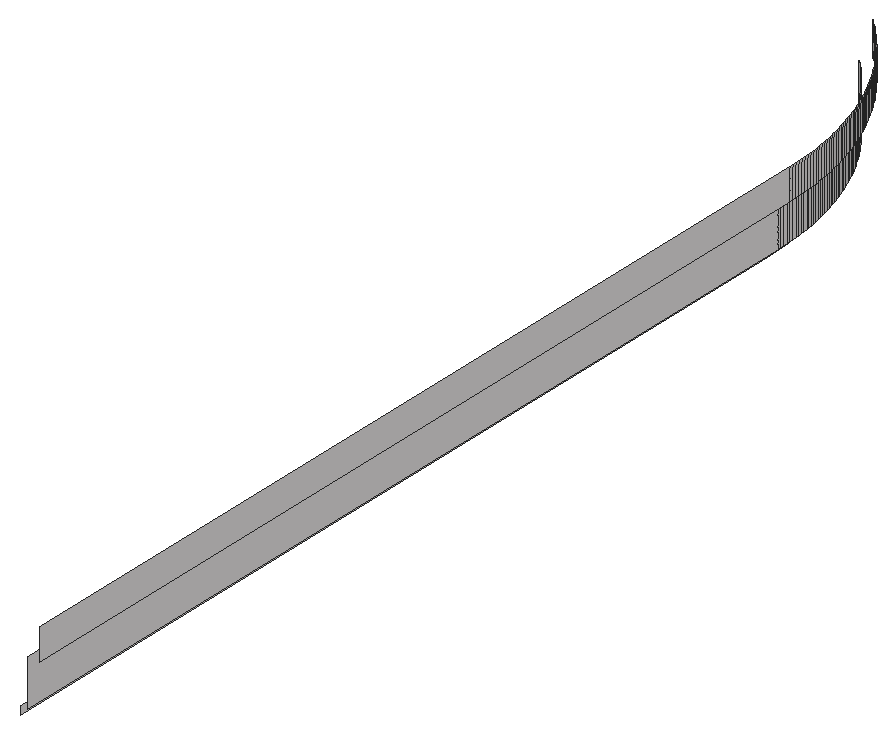
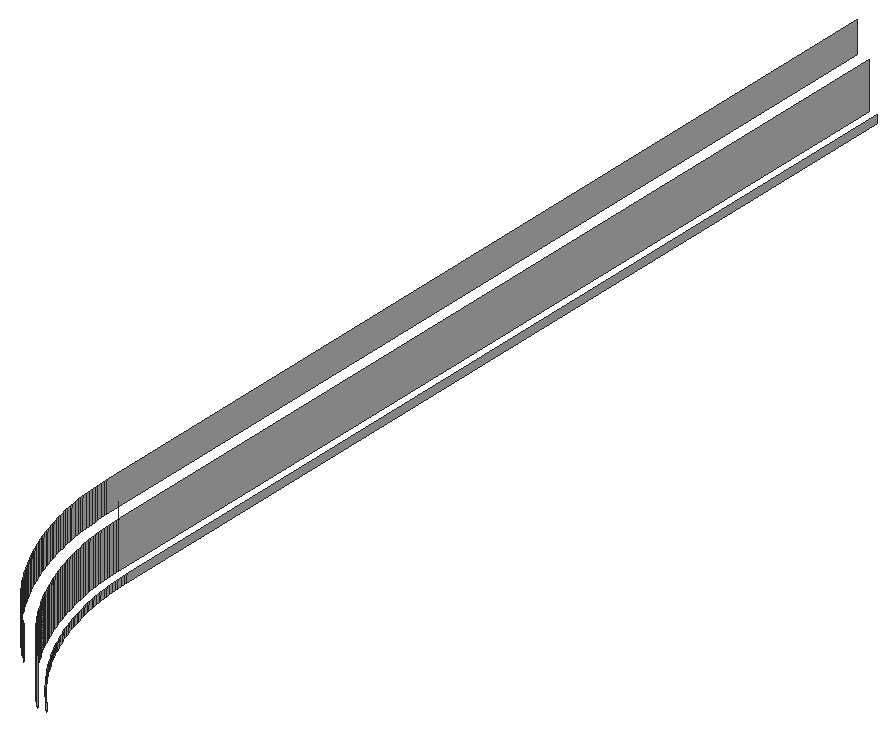
# SketchUp Ruby script. Lengths in inches.
U = 1.inch
M = Sketchup.active_model
def pt(a) = Geom::Point3d.new(a.map { |v| v * U })
def face(e, loops, mat)
  f = e.add_face(loops[0].map { |a| pt(a) })
  loops[1..].each { |l| e.add_face(l.map { |a| pt(a) }).erase! }
  f.material = f.back_material = mat if mat
  f
end
# faces: each face lists its corners as indices into pts; further lists are holes
def faces(e, pts, list, mat = nil) = list.each { |f| face(e, (f[0].is_a?(Array) ? f : [f]).map { |l| l.map { |i| pts[i] } }, mat) }
# xy, xz, yz: faces in a plane at the given z, y or x. An outline is a flat list of corners, or four numbers for a rectangle; further outlines are holes
def ring(l) = l.size == 4 ? [[l[0], l[1]], [l[2], l[1]], [l[2], l[3]], [l[0], l[3]]] : l.each_slice(2).to_a
def flat(e, list, mat, &to3) = list.each { |f| face(e, (f[0].is_a?(Array) ? f : [f]).map { |l| ring(l).map { |u, v| to3.(u, v) } }, mat) }
def xy(e, z, list, mat = nil) = flat(e, list, mat) { |x, y| [x, y, z] }
def xz(e, y, list, mat = nil) = flat(e, list, mat) { |x, z| [x, y, z] }
def yz(e, x, list, mat = nil) = flat(e, list, mat) { |y, z| [x, y, z] }
def lines(e, pts, list) = list.each { |a, b| e.add_line(pt(pts[a]), pt(pts[b])) }
# prism: a flat outline (further loops are holes) pulled along v
def prism(e, loops, v, mat = nil)
  f = face(e, loops, mat); d = Geom::Vector3d.new(v.map { |x| x * U })
  f.pushpull(f.normal.samedirection?(d) ? d.length : -d.length)
end
def box(e, o, s, mat = nil) = prism(e, [[o, [o[0] + s[0], o[1], o[2]], [o[0] + s[0], o[1] + s[1], o[2]], [o[0], o[1] + s[1], o[2]]]], [0, 0, s[2]], mat)
def at(x, y, z, deg = 0) = Geom::Transformation.translation(pt([x, y, z])) * Geom::Transformation.rotation(ORIGIN, Z_AXIS, deg.degrees)
def axes(o, x, y, z) = Geom::Transformation.new([*x, 0, *y, 0, *z, 0, *pt(o).to_a, 1])
def part(name) = M.definitions.add(name)
# library, detail: a bought-in or finely detailed component or shape, given as its bounding box
def library(name, o, s) = part(name).tap { |d| box(d.entities, o, s) }
def detail(e, o, s) = box(e.add_group.entities, o, s)
def put(e, d, t, mat = nil) = e.add_instance(d, t).tap { |i| i.material = mat if mat }
def group(e, t, mat = nil) = e.add_group.tap { |g| g.transformation = t; g.material = mat if mat }.entities
root = M.entities
M.materials.add("[Quartz Light Brown]").color = [215, 212, 212]
yz(root,501,[[320.7,486,440.7,487],[440.7,486,441.19,487]],"[Quartz Light Brown]")
yz(root,502,[[320.7,487,440.7,493],[440.7,487,441.2,493]],"[Quartz Light Brown]")
yz(root,503.5,[[320.7,493,440.7,497],[440.7,493,441.22,497]],"[Quartz Light Brown]")
p = [[501,441.19,486],[500.99,441.67,486],[500.99,441.67,487],[501,441.19,487],[500.97,442.15,486],[500.97,442.15,487],
  [500.95,442.64,486],[500.95,442.64,487],[500.92,443.12,486],[500.92,443.12,487],[500.89,443.6,486],[500.89,443.6,487],
  [500.84,444.09,486],[500.84,444.09,487],[500.8,444.57,486],[500.8,444.57,487],[500.74,445.05,486],[500.74,445.05,487],
  [500.68,445.53,486],[500.68,445.53,487],[500.62,446.01,486],[500.62,446.01,487],[500.54,446.49,486],[500.54,446.49,487],
  [500.47,446.97,486],[500.47,446.97,487],[500.38,447.44,486],[500.38,447.44,487],[500.29,447.92,486],[500.29,447.92,487],
  [500.19,448.39,486],[500.19,448.39,487],[500.09,448.87,486],[500.09,448.87,487],[499.98,449.34,486],[499.98,449.34,487],
  [499.86,449.81,486],[499.86,449.81,487],[499.74,450.28,486],[499.74,450.28,487],[499.61,450.74,486],[499.61,450.74,487],
  [499.48,451.21,486],[499.48,451.21,487],[499.34,451.67,486],[499.34,451.67,487],[499.1875,452.13,486],[499.1875,452.13,487],
  [499.04,452.59,486],[499.04,452.59,487],[498.88,453.05,486],[498.88,453.05,487],[498.71,453.51,486],[498.71,453.51,487],
  [498.54,453.96,486],[498.54,453.96,487],[498.37,454.41,486],[498.37,454.41,487],[498.18,454.86,486],[498.18,454.86,487],
  [498,455.31,486],[498,455.31,487],[497.8,455.75,486],[497.8,455.75,487],[497.6,456.19,486],[497.6,456.19,487],
  [497.4,456.63,486],[497.4,456.63,487],[497.18,457.07,486],[497.18,457.07,487],[496.97,457.5,486],[496.97,457.5,487],
  [496.74,457.93,486],[496.74,457.93,487],[496.52,458.36,486],[496.52,458.36,487],[496.28,458.78,486],[496.28,458.78,487],
  [496.04,459.2,486],[496.04,459.2,487],[495.8,459.62,486],[495.8,459.62,487],[495.55,460.03,486],[495.55,460.03,487],
  [495.29,460.44,486],[495.29,460.44,487],[495.03,460.85,486],[495.03,460.85,487],[494.76,461.26,486],[494.76,461.26,487],
  [494.49,461.66,486],[494.49,461.66,487],[494.22,462.06,486],[494.22,462.06,487],[493.93,462.45,486],[493.93,462.45,487],
  [493.65,462.84,486],[493.65,462.84,487],[493.35,463.23,486],[493.35,463.23,487],[493.06,463.61,486],[493.06,463.61,487],
  [492.75,463.99,486],[492.75,463.99,487],[492.45,464.36,486],[492.45,464.36,487],[492.14,464.73,486],[492.14,464.73,487],
  [491.82,465.1,486],[491.82,465.1,487],[491.5,465.46,486],[491.5,465.46,487],[491.17,465.82,486],[491.17,465.82,487],
  [490.84,466.17,486],[490.84,466.17,487],[501.99,441.7,487],[501.99,441.7,493],[502,441.2,493],[502,441.2,487],
  [501.97,442.19,487],[501.97,442.19,493],[501.95,442.69,487],[501.95,442.69,493],[501.92,443.1875,487],[501.92,443.1875,493],
  [501.88,443.68,487],[501.88,443.68,493],[501.84,444.18,487],[501.84,444.18,493],[501.79,444.67,487],[501.79,444.67,493],
  [501.74,445.17,487],[501.74,445.17,493],[501.67,445.66,487],[501.67,445.66,493],[501.61,446.15,487],[501.61,446.15,493],
  [501.53,446.65,487],[501.53,446.65,493],[501.45,447.14,487],[501.45,447.14,493],[501.36,447.625,487],[501.36,447.625,493],
  [501.27,448.11,487],[501.27,448.11,493],[501.17,448.6,487],[501.17,448.6,493],[501.0625,449.09,487],[501.0625,449.09,493],
  [500.95,449.57,487],[500.95,449.57,493],[500.83,450.05,487],[500.83,450.05,493],[500.71,450.54,487],[500.71,450.54,493],
  [500.57,451.02,487],[500.57,451.02,493],[500.44,451.49,487],[500.44,451.49,493],[500.29,451.97,487],[500.29,451.97,493],
  [500.14,452.44,487],[500.14,452.44,493],[499.98,452.92,487],[499.98,452.92,493],[499.82,453.39,487],[499.82,453.39,493],
  [499.65,453.85,487],[499.65,453.85,493],[499.48,454.32,487],[499.48,454.32,493],[499.29,454.78,487],[499.29,454.78,493],
  [499.11,455.24,487],[499.11,455.24,493],[498.91,455.7,487],[498.91,455.7,493],[498.71,456.16,487],[498.71,456.16,493],
  [498.51,456.61,487],[498.51,456.61,493],[498.3,457.06,487],[498.3,457.06,493],[498.08,457.51,487],[498.08,457.51,493],
  [497.86,457.95,487],[497.86,457.95,493],[497.63,458.39,487],[497.63,458.39,493],[497.4,458.83,487],[497.4,458.83,493],
  [497.15,459.27,487],[497.15,459.27,493],[496.91,459.7,487],[496.91,459.7,493],[496.66,460.13,487],[496.66,460.13,493],
  [496.4,460.56,487],[496.4,460.56,493],[496.14,460.98,487],[496.14,460.98,493],[495.87,461.4,487],[495.87,461.4,493],
  [495.6,461.8125,487],[495.6,461.8125,493],[495.32,462.22,487],[495.32,462.22,493],[495.03,462.63,487],[495.03,462.63,493],
  [494.74,463.04,487],[494.74,463.04,493],[494.45,463.4375,487],[494.45,463.4375,493],[494.15,463.83,487],[494.15,463.83,493],
  [493.84,464.23,487],[493.84,464.23,493],[493.53,464.62,487],[493.53,464.62,493],[493.22,465,487],[493.22,465,493],
  [492.9,465.38,487],[492.9,465.38,493],[492.57,465.76,487],[492.57,465.76,493],[492.24,466.13,487],[492.24,466.13,493],
  [491.9,466.5,487],[491.9,466.5,493],[491.5625,466.86,487],[491.5625,466.86,493],[491.22,467.22,487],[491.22,467.22,493],
  [490.87,467.57,487],[490.87,467.57,493],[503.5,441.22,493],[503.49,441.73,493],[503.49,441.73,497],[503.5,441.22,497],
  [503.47,442.25,493],[503.47,442.25,497],[503.45,442.77,493],[503.45,442.77,497],[503.42,443.28,493],[503.42,443.28,497],
  [503.38,443.8,493],[503.38,443.8,497],[503.33,444.32,493],[503.33,444.32,497],[503.28,444.83,493],[503.28,444.83,497],
  [503.23,445.34,493],[503.23,445.34,497],[503.16,445.86,493],[503.16,445.86,497],[503.09,446.37,493],[503.09,446.37,497],
  [503.01,446.88,493],[503.01,446.88,497],[502.93,447.39,493],[502.93,447.39,497],[502.84,447.9,493],[502.84,447.9,497],
  [502.74,448.41,493],[502.74,448.41,497],[502.64,448.91,493],[502.64,448.91,497],[502.53,449.42,493],[502.53,449.42,497],
  [502.41,449.92,493],[502.41,449.92,497],[502.28,450.42,493],[502.28,450.42,497],[502.15,450.92,493],[502.15,450.92,497],
  [502.02,451.42,493],[502.02,451.42,497],[501.875,451.92,493],[501.875,451.92,497],[501.72,452.41,493],[501.72,452.41,497],
  [501.57,452.91,493],[501.57,452.91,497],[501.4,453.4,493],[501.4,453.4,497],[501.23,453.89,493],[501.23,453.89,497],
  [501.06,454.37,493],[501.06,454.37,497],[500.875,454.86,493],[500.875,454.86,497],[500.6875,455.34,493],[500.6875,455.34,497],
  [500.49,455.82,493],[500.49,455.82,497],[500.29,456.29,493],[500.29,456.29,497],[500.09,456.77,493],[500.09,456.77,497],
  [499.87,457.24,493],[499.87,457.24,497],[499.65,457.71,493],[499.65,457.71,497],[499.43,458.17,493],[499.43,458.17,497],
  [499.19,458.63,493],[499.19,458.63,497],[498.96,459.09,493],[498.96,459.09,497],[498.71,459.55,493],[498.71,459.55,497],
  [498.46,460,493],[498.46,460,497],[498.21,460.45,493],[498.21,460.45,497],[497.95,460.9,493],[497.95,460.9,497],
  [497.68,461.34,493],[497.68,461.34,497],[497.41,461.78,493],[497.41,461.78,497],[497.13,462.21,493],[497.13,462.21,497],
  [496.84,462.65,493],[496.84,462.65,497],[496.55,463.07,493],[496.55,463.07,497],[496.26,463.5,493],[496.26,463.5,497],
  [495.96,463.92,493],[495.96,463.92,497],[495.65,464.33,493],[495.65,464.33,497],[495.34,464.75,493],[495.34,464.75,497],
  [495.02,465.16,493],[495.02,465.16,497],[494.7,465.56,493],[494.7,465.56,497],[494.37,465.96,493],[494.37,465.96,497],
  [494.04,466.35,493],[494.04,466.35,497],[493.7,466.75,493],[493.7,466.75,497],[493.35,467.13,493],[493.35,467.13,497],
  [493.01,467.51,493],[493.01,467.51,497],[492.65,467.89,493],[492.65,467.89,497],[492.29,468.26,493],[492.29,468.26,497],
  [491.93,468.63,493],[491.93,468.63,497],[491.5625,468.99,493],[491.5625,468.99,497],[491.19,469.35,493],[491.19,469.35,497],
  [502,440.7,493],[502,440.7,495]]
faces(root,p,[[0,1,2,3],[1,4,5,2],[4,6,7,5],[6,8,9,7],[8,10,11,9],[10,12,13,11],[12,14,15,13],[14,16,17,15],
  [16,18,19,17],[18,20,21,19],[20,22,23,21],[22,24,25,23],[24,26,27,25],[26,28,29,27],[28,30,31,29],[30,32,33,31],
  [32,34,35,33],[34,36,37,35],[36,38,39,37],[38,40,41,39],[40,42,43,41],[42,44,45,43],[44,46,47,45],[46,48,49,47],
  [48,50,51,49],[50,52,53,51],[52,54,55,53],[54,56,57,55],[56,58,59,57],[58,60,61,59],[60,62,63,61],[62,64,65,63],
  [64,66,67,65],[66,68,69,67],[68,70,71,69],[70,72,73,71],[72,74,75,73],[74,76,77,75],[76,78,79,77],[78,80,81,79],
  [80,82,83,81],[82,84,85,83],[84,86,87,85],[86,88,89,87],[88,90,91,89],[90,92,93,91],[92,94,95,93],[94,96,97,95],
  [96,98,99,97],[98,100,101,99],[100,102,103,101],[102,104,105,103],[104,106,107,105],[106,108,109,107],[108,110,111,109],[110,112,113,111],
  [112,114,115,113],[116,117,118,119],[120,121,117,116],[122,123,121,120],[124,125,123,122],[126,127,125,124],[128,129,127,126],[130,131,129,128],
  [132,133,131,130],[134,135,133,132],[136,137,135,134],[138,139,137,136],[140,141,139,138],[142,143,141,140],[144,145,143,142],[146,147,145,144],
  [148,149,147,146],[150,151,149,148],[152,153,151,150],[154,155,153,152],[156,157,155,154],[158,159,157,156],[160,161,159,158],[162,163,161,160],
  [164,165,163,162],[166,167,165,164],[168,169,167,166],[170,171,169,168],[172,173,171,170],[174,175,173,172],[176,177,175,174],[178,179,177,176],
  [180,181,179,178],[182,183,181,180],[184,185,183,182],[186,187,185,184],[188,189,187,186],[190,191,189,188],[192,193,191,190],[194,195,193,192],
  [196,197,195,194],[198,199,197,196],[200,201,199,198],[202,203,201,200],[204,205,203,202],[206,207,205,204],[208,209,207,206],[210,211,209,208],
  [212,213,211,210],[214,215,213,212],[216,217,215,214],[218,219,217,216],[220,221,219,218],[222,223,221,220],[224,225,223,222],[226,227,225,224],
  [228,229,227,226],[230,231,229,228],[232,233,231,230],[234,235,233,232],[236,237,238,239],[237,240,241,238],[240,242,243,241],[242,244,245,243],
  [244,246,247,245],[246,248,249,247],[248,250,251,249],[250,252,253,251],[252,254,255,253],[254,256,257,255],[256,258,259,257],[258,260,261,259],
  [260,262,263,261],[262,264,265,263],[264,266,267,265],[266,268,269,267],[268,270,271,269],[270,272,273,271],[272,274,275,273],[274,276,277,275],
  [276,278,279,277],[278,280,281,279],[280,282,283,281],[282,284,285,283],[284,286,287,285],[286,288,289,287],[288,290,291,289],[290,292,293,291],
  [292,294,295,293],[294,296,297,295],[296,298,299,297],[298,300,301,299],[300,302,303,301],[302,304,305,303],[304,306,307,305],[306,308,309,307],
  [308,310,311,309],[310,312,313,311],[312,314,315,313],[314,316,317,315],[316,318,319,317],[318,320,321,319],[320,322,323,321],[322,324,325,323],
  [324,326,327,325],[326,328,329,327],[328,330,331,329],[330,332,333,331],[332,334,335,333],[334,336,337,335],[336,338,339,337],[338,340,341,339],
  [340,342,343,341],[342,344,345,343],[344,346,347,345],[346,348,349,347],[348,350,351,349],[350,352,353,351],[352,354,355,353],[354,356,357,355],
  [356,358,359,357]],"[Quartz Light Brown]")
lines(root,p,[[360,361]])
